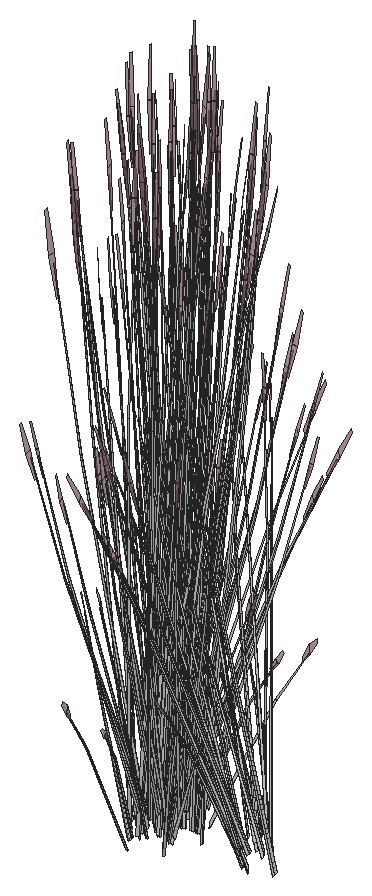
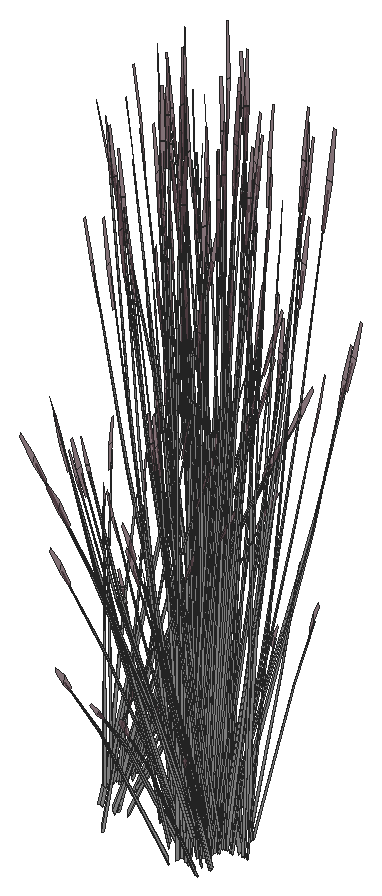
# SketchUp Ruby script. Lengths in inches.
U = 1.inch
M = Sketchup.active_model
def pt(a) = Geom::Point3d.new(a.map { |v| v * U })
def face(e, loops, mat)
  f = e.add_face(loops[0].map { |a| pt(a) })
  loops[1..].each { |l| e.add_face(l.map { |a| pt(a) }).erase! }
  f.material = f.back_material = mat if mat
  f
end
# faces: each face lists its corners as indices into pts; further lists are holes
def faces(e, pts, list, mat = nil) = list.each { |f| face(e, (f[0].is_a?(Array) ? f : [f]).map { |l| l.map { |i| pts[i] } }, mat) }
# xy, xz, yz: faces in a plane at the given z, y or x. An outline is a flat list of corners, or four numbers for a rectangle; further outlines are holes
def ring(l) = l.size == 4 ? [[l[0], l[1]], [l[2], l[1]], [l[2], l[3]], [l[0], l[3]]] : l.each_slice(2).to_a
def flat(e, list, mat, &to3) = list.each { |f| face(e, (f[0].is_a?(Array) ? f : [f]).map { |l| ring(l).map { |u, v| to3.(u, v) } }, mat) }
def xy(e, z, list, mat = nil) = flat(e, list, mat) { |x, y| [x, y, z] }
def xz(e, y, list, mat = nil) = flat(e, list, mat) { |x, z| [x, y, z] }
def yz(e, x, list, mat = nil) = flat(e, list, mat) { |y, z| [x, y, z] }
def lines(e, pts, list) = list.each { |a, b| e.add_line(pt(pts[a]), pt(pts[b])) }
# prism: a flat outline (further loops are holes) pulled along v
def prism(e, loops, v, mat = nil)
  f = face(e, loops, mat); d = Geom::Vector3d.new(v.map { |x| x * U })
  f.pushpull(f.normal.samedirection?(d) ? d.length : -d.length)
end
def box(e, o, s, mat = nil) = prism(e, [[o, [o[0] + s[0], o[1], o[2]], [o[0] + s[0], o[1] + s[1], o[2]], [o[0], o[1] + s[1], o[2]]]], [0, 0, s[2]], mat)
def at(x, y, z, deg = 0) = Geom::Transformation.translation(pt([x, y, z])) * Geom::Transformation.rotation(ORIGIN, Z_AXIS, deg.degrees)
def axes(o, x, y, z) = Geom::Transformation.new([*x, 0, *y, 0, *z, 0, *pt(o).to_a, 1])
def part(name) = M.definitions.add(name)
# library, detail: a bought-in or finely detailed component or shape, given as its bounding box
def library(name, o, s) = part(name).tap { |d| box(d.entities, o, s) }
def detail(e, o, s) = box(e.add_group.entities, o, s)
def put(e, d, t, mat = nil) = e.add_instance(d, t).tap { |i| i.material = mat if mat }
def group(e, t, mat = nil) = e.add_group.tap { |g| g.transformation = t; g.material = mat if mat }.entities
root = M.entities
M.materials.add("LightPink_Translucent").color = [144, 107, 117]
M.materials["LightPink_Translucent"].alpha = 0.75
M.materials.add("[_0053_Ivory_]").color = [200, 200, 200]
c1 = part("blade")
p = [[2.15,0.21,22],[0,0.17,0],[0.09,0.45,0],[2.18,0.31,22],[2.29,0.31,22],[0.38,0.45,0],
  [2.48,0.24,33],[2.49,0.24,33],[2.48,0.22,33]]
faces(c1.entities,p,[[0,1,2,3],[4,5,2,3],[6,3,4,7],[8,0,3,6]])
c2 = part("seeds")
p = [[0.3,-0.1,1.38],[-0.01,-0.03,1.59],[-0.01,-0.03,0.03],[0.14,-0.07,-0.07],[0.29,-0.03,3],[0.15,0.01,3.11]]
faces(c2.entities,p,[[0,1,2,3],[1,0,4,5]],"LightPink_Translucent")
c3 = part("blade with seeds")
put(c3.entities,c1,at(0,0,0))
put(c3.entities,c2,axes([2.4,0.25,30.99],[1.5799,-0.05474,1.17369],[-0.12525,1.92788,0.29478],[-0.07173,-0.02425,1.56792]))
put(root,c3,axes([458.04,103.93,128.86],[-0.36485,-0.52782,-0.44739],[0.55265,-0.37168,0.21531],[-0.11807,-0.06531,1.43643]),"[_0053_Ivory_]")
put(root,c3,axes([457.01,105.32,131.99],[-0.0158,0.58168,-0.7886],[-0.66548,-0.03907,0.09517],[-0.07023,0.24643,1.11556]),"[_0053_Ivory_]")
put(root,c3,axes([456.99,106.96,129.42],[-0.01572,-0.37392,1.1486],[0.39276,0.26669,0.84392],[-0.07724,0.17822,0.25299]),"[_0053_Ivory_]")
put(root,c3,axes([458.82,104.31,128.86],[-0.65953,0.03882,-0.44739],[-0.05964,-0.64439,0.21531],[-0.11807,0.06531,1.43643]),"[_0053_Ivory_]")
put(root,c3,axes([457.56,105.39,129.13],[0.56842,0.31443,0.49651],[-0.33976,0.56381,0],[-0.12946,-0.07161,1.57504]),"[_0053_Ivory_]")
put(root,c3,axes([456.78,106.14,130.02],[0.01334,-0.32463,1.54345],[0.60018,0.17147,0.21329],[-0.052,0.34598,0.72882]),"[_0053_Ivory_]")
put(root,c3,axes([458.09,104.23,129.09],[0.16098,-0.74515,-0.23429],[0.76326,0.12989,0.51271],[-0.13337,-0.1029,1.5644]),"[_0053_Ivory_]")
put(root,c3,axes([458.37,104.41,129.27],[-0.11717,0.56122,0.1448],[-0.57245,-0.09742,-0.41347],[-0.10418,-0.05763,1.26744]),"[_0053_Ivory_]")
put(root,c3,axes([459.51,105.97,128.67],[-0.56842,0.31443,-0.49651],[-0.33976,-0.56381,0],[-0.12946,0.07161,1.57504]),"[_0053_Ivory_]")
put(root,c3,axes([456.14,102.84,128.67],[0,-0.62885,-0.49651],[0.67951,0,0],[0,-0.14322,1.57504]),"[_0053_Ivory_]")
put(root,c3,axes([456.44,103.42,129.13],[0,0.62885,0.49651],[-0.67951,0,0],[0,-0.14322,1.57504]),"[_0053_Ivory_]")
put(root,c3,axes([459.55,105.8,128.85],[-0.37499,-0.63235,-0.05142],[0.6353,-0.35142,0.51607],[-0.15655,0.0602,1.6363]),"[_0053_Ivory_]")
put(root,c3,axes([457.14,105.52,131.66],[0.43478,0.42253,-0.5672],[-0.45929,0.37004,-0.43934],[-0.06615,0.21468,1.08528]),"[_0053_Ivory_]")
put(root,c3,axes([459.375,105.72,128.68],[-0.56663,-0.1556,-0.30978],[0.14267,-0.54795,0.30978],[-0.11423,0.06319,1.38974]),"[_0053_Ivory_]")
put(root,c3,axes([457.92,103.57,129.32],[-0.68399,-0.30005,-0.29095],[0.32934,-0.63331,-0.50002],[-0.0215,-0.15549,1.59708]),"[_0053_Ivory_]")
put(root,c3,axes([459.7,103.38,129.5],[-0.01659,-0.59209,1.41272],[0.75089,0.15348,0.59816],[-0.1776,0.32398,1.3335]),"[_0053_Ivory_]")
put(root,c3,axes([456.67,106.15,129.48],[0.55175,-0.11136,0.06507],[0.12684,0.44864,-0.86304],[-0.03498,0.22711,0.7736]),"[_0053_Ivory_]")
put(root,c3,axes([459.28,104.13,129.32],[0.07077,0.71755,-0.29095],[-0.73712,0.04339,-0.50002],[-0.1298,0.09558,1.59708]),"[_0053_Ivory_]")
put(root,c3,axes([457.61,102.93,128.75],[-0.24943,-0.64486,-0.69835],[0.71849,-0.23224,-0.18329],[-0.02757,-0.21836,1.54149]),"[_0053_Ivory_]")
put(root,c3,axes([458.74,100.91,131.33],[-0.59704,-0.15764,-0.51099],[0.20464,-0.54049,-0.3958],[-0.05475,-0.21761,0.97773]),"[_0053_Ivory_]")
put(root,c3,axes([457.64,104.91,130.53],[-0.01487,-0.24136,1.71376],[0.64429,0.16012,0.13857],[-0.03985,0.34396,0.73262]),"[_0053_Ivory_]")
put(root,c3,axes([456.4375,102.85,128.68],[0.42396,-0.39235,-0.30978],[0.42396,0.39235,0.30978],[0,-0.12637,1.38974]),"[_0053_Ivory_]")
put(root,c3,axes([458.35,100.32,128.78],[-0.4197,0.36076,-0.03893],[-0.38456,-0.39511,-0.17649],[-0.02707,-0.11196,0.58215]),"[_0053_Ivory_]")
put(root,c3,axes([458.18,103.875,129.01],[0.76764,0.13249,0.45755],[-0.15622,0.74829,0.17955],[-0.11218,-0.07226,1.58856]),"[_0053_Ivory_]")
put(root,c3,axes([457.98,103.74,129.37],[-0.29468,0.56664,0.44739],[-0.61229,-0.27271,-0.21531],[0,-0.13062,1.43643]),"[_0053_Ivory_]")
put(root,c3,axes([458.95,101.01,131.63],[-0.28988,-0.51132,-0.71045],[0.59671,-0.28496,0.08574],[-0.06778,-0.24706,1.00501]),"[_0053_Ivory_]")
put(root,c3,axes([457.77,105.07,129.13],[0.65264,-0.16691,0.17642],[0.16115,0.62115,0.35086],[-0.05821,-0.0905,1.60407]),"[_0053_Ivory_]")
put(root,c3,axes([458.61,105.17,128.85],[-0.61229,-0.28233,0],[0.29468,-0.58663,0],[0,0,1.62707]),"[_0053_Ivory_]")
put(root,c3,axes([460.03,105.875,129.03],[0.37973,0.63014,0],[-0.6353,0.35142,-0.51607],[-0.14469,0.08004,1.63711]),"[_0053_Ivory_]")
put(root,c3,axes([459.71,105.1,129.13],[0.17545,-0.62497,0.17642],[0.64204,0.17686,0.35086],[-0.11091,0.00304,1.60407]),"[_0053_Ivory_]")
put(root,c3,axes([459.41,104.27,129.27],[0.44871,0.37783,0.1448],[-0.37428,0.42627,-0.41347],[-0.10418,0.05763,1.26744]),"[_0053_Ivory_]")
put(root,c3,axes([459.25,103.81,128.95],[-0.56493,-0.54126,-0.06131],[0.56528,-0.54159,0],[-0.01973,-0.0189,1.75571]),"[_0053_Ivory_]")
put(root,c3,axes([459.4,104,129.37],[0.65953,-0.03882,0.44739],[0.05964,0.64439,-0.21531],[-0.11807,0.06531,1.43643]),"[_0053_Ivory_]")
put(root,c3,axes([459.5625,105.48,128.98],[0.76036,0.2044,0.30756],[-0.19023,0.7306,-0.36492],[-0.12585,0.09144,1.64885]),"[_0053_Ivory_]")
put(root,c3,axes([458.45,99.875,128.15],[-0.10187,0.02266,1.76342],[-0.56336,-0.25503,-0.26939],[0.00945,-0.21273,0.30037]),"[_0053_Ivory_]")
put(root,c3,axes([459.89,105.4375,129.13],[0.56842,-0.31443,0.49651],[0.33976,0.56381,0],[-0.12946,0.07161,1.57504]),"[_0053_Ivory_]")
put(root,c3,axes([459.01,100.57,131.18],[0.1831,-0.48359,-0.35414],[0.53419,0.14105,0.4572],[-0.04898,-0.1947,0.87481]),"[_0053_Ivory_]")
put(root,c3,axes([458.12,103.18,129.01],[0.26406,0.70318,0.45755],[-0.7545,0.24452,0.17955],[0.00922,-0.12921,1.58856]),"[_0053_Ivory_]")
put(root,c3,axes([457.99,103.1,128.86],[0.29468,-0.56664,-0.44739],[0.61229,0.27271,0.21531],[0,-0.13062,1.43643]),"[_0053_Ivory_]")
put(root,c3,axes([458.75,104.92,128.86],[-0.19817,-0.54216,0],[0.56587,-0.18986,0],[0,0,1.54371]),"[_0053_Ivory_]")
put(root,c3,axes([458.03,106.07,128.15],[0.09829,-0.03422,1.76342],[0.59126,0.18834,-0.26939],[0.01729,0.21228,0.30037]),"[_0053_Ivory_]")
put(root,c3,axes([458.16,106.26,131.18],[-0.1831,0.48359,-0.35414],[-0.53419,-0.14105,0.4572],[0.04898,0.1947,0.87481]),"[_0053_Ivory_]")
put(root,c3,axes([459.55,103.85,128.86],[-0.29468,0.56664,-0.44739],[-0.61229,-0.27271,0.21531],[0,0.13062,1.43643]),"[_0053_Ivory_]")
put(root,c3,axes([460.71,103.51,129.13],[-0.47719,-0.45806,0.17642],[0.48088,-0.44429,0.35086],[-0.0527,0.09355,1.60407]),"[_0053_Ivory_]")
put(root,c3,axes([459.06,103.24,128.86],[0,-0.72763,0],[0.75945,0,0],[0,0,1.79456]),"[_0053_Ivory_]")
put(root,c3,axes([458.36,103.375,129.09],[0.68433,0.30479,0.24065],[-0.32934,0.63331,0.50002],[0,-0.14599,1.60543]),"[_0053_Ivory_]")
put(root,c3,axes([459.45,103.53,128.95],[0,0.72727,-0.05637],[-0.75945,0,0],[0,0.02286,1.79368]),"[_0053_Ivory_]")
put(root,c3,axes([458.14,102.95,129.37],[-0.65953,0.03882,0.44739],[-0.05964,-0.64439,-0.21531],[0.11807,-0.06531,1.43643]),"[_0053_Ivory_]")
put(root,c3,axes([457.83,101.85,129.13],[-0.17545,0.62497,0.17642],[-0.64204,-0.17686,0.35086],[0.11091,-0.00304,1.60407]),"[_0053_Ivory_]")
put(root,c3,axes([459.08,104.94,128.94],[0.26406,0.72244,-0.06012],[-0.7545,0.25315,0],[0.00922,0.02523,1.72173]),"[_0053_Ivory_]")
put(root,c3,axes([457.52,101.07,129.03],[-0.37973,-0.63014,0],[0.6353,-0.35142,-0.51607],[0.14469,-0.08004,1.63711]),"[_0053_Ivory_]")
put(root,c3,axes([458.21,105.82,131.63],[0.28988,0.51132,-0.71045],[-0.59671,0.28496,0.08574],[0.06778,0.24706,1.00501]),"[_0053_Ivory_]")
put(root,c3,axes([461.26,103.99,128.85],[-0.75908,-0.00503,-0.04976],[0,-0.70283,0.49943],[-0.02386,0.16,1.58352]),"[_0053_Ivory_]")
put(root,c3,axes([459.77,101.88,129.13],[-0.65264,0.16691,0.17642],[-0.16115,-0.62115,0.35086],[0.05821,0.0905,1.60407]),"[_0053_Ivory_]")
put(root,c3,axes([459.11,99.55,129.42],[0.07791,0.3667,1.1486],[-0.43222,-0.2031,0.84392],[0.04651,-0.18776,0.25299]),"[_0053_Ivory_]")
put(root,c3,axes([458.7,102.79,129.01],[-0.50358,0.57069,0.45755],[-0.59827,-0.50377,0.17955],[0.1214,-0.05695,1.58856]),"[_0053_Ivory_]")
put(root,c3,axes([459.57,103.6875,128.87],[0.42396,0.40619,0],[-0.42396,0.40619,0],[0,0,1.69266]),"[_0053_Ivory_]")
put(root,c3,axes([459.56,103.21,129.37],[0.29468,-0.56664,0.44739],[0.61229,0.27271,-0.21531],[0,0.13062,1.43643]),"[_0053_Ivory_]")
put(root,c3,axes([459.3,105.18,128.86],[0.61229,0.28233,0],[-0.29468,0.58663,0],[0,0,1.74954]),"[_0053_Ivory_]")
put(root,c3,axes([458.43,105.93,131.33],[0.59704,0.15764,-0.51099],[-0.20464,0.54049,-0.3958],[0.05475,0.21761,0.97773]),"[_0053_Ivory_]")
put(root,c3,axes([459.36,103.08,129.03],[-0.76764,-0.13249,0.49198],[0.15622,-0.74829,0.19306],[0.11218,0.07226,1.70813]),"[_0053_Ivory_]")
put(root,c3,axes([461.11,104.1,128.68],[-0.42396,0.39235,-0.30978],[-0.42396,-0.39235,0.30978],[0,0.12637,1.38974]),"[_0053_Ivory_]")
put(root,c3,axes([459.89,104.02,128.75],[0.2227,0.57576,-0.69212],[-0.64151,0.20736,-0.18165],[0.02462,0.19497,1.52773]),"[_0053_Ivory_]")
put(root,c3,axes([459.58,103.41,128.86],[0.67951,0,0],[0,0.65103,0],[0,0,1.78407]),"[_0053_Ivory_]")
put(root,c3,axes([458.93,102.6875,129.37],[-0.36485,-0.52782,0.44739],[0.55265,-0.37168,-0.21531],[0.11807,0.06531,1.43643]),"[_0053_Ivory_]")
put(root,c3,axes([458.26,102.8125,129.32],[-0.07077,-0.71755,-0.29095],[0.73712,-0.04339,-0.50002],[0.1298,-0.09558,1.59708]),"[_0053_Ivory_]")
put(root,c3,axes([459.82,103.34,129.27],[0.56587,-0.18339,0.1448],[0.19817,0.52368,-0.41347],[0,0.11525,1.26744]),"[_0053_Ivory_]")
put(root,c3,axes([460.03,101.31,131.33],[-0.43478,-0.42253,-0.51099],[0.45929,-0.37004,-0.3958],[0.06615,-0.21468,0.97773]),"[_0053_Ivory_]")
put(root,c3,axes([459.62,103.38,129.32],[0.68399,0.30005,-0.29095],[-0.32934,0.63331,-0.50002],[0.0215,0.15549,1.59708]),"[_0053_Ivory_]")
put(root,c3,axes([458.17,101.23,128.68],[0.56663,0.1556,-0.30978],[-0.14267,0.54795,0.30978],[0.11423,-0.06319,1.38974]),"[_0053_Ivory_]")
put(root,c3,axes([459.74,100.57,129.24],[-0.17264,0.12729,1.43002],[-0.51703,-0.22279,-0.30754],[0.09584,-0.27707,0.61141]),"[_0053_Ivory_]")
put(root,c3,axes([467.35,101.62,130.53],[0.25192,-0.01424,1.71376],[-0.16712,0.61729,0.13857],[-0.35901,-0.03818,0.73262]),"[_0053_Ivory_]")
put(root,c3,axes([461.11,103.53,129.13],[0,-0.62885,0.49651],[0.67951,0,0],[0,0.14322,1.57504]),"[_0053_Ivory_]")
put(root,c3,axes([461.4,104.11,128.67],[0,0.62885,-0.49651],[-0.67951,0,0],[0,0.14322,1.57504]),"[_0053_Ivory_]")
put(root,c3,axes([458.03,100.98,128.67],[0.56842,-0.31443,-0.49651],[0.33976,0.56381,0],[0.12946,-0.07161,1.57504]),"[_0053_Ivory_]")
put(root,c3,axes([458.77,104.8125,130.53],[-0.13883,-0.2019,1.71376],[0.64153,-0.16998,0.13857],[0.14499,0.31697,0.73262]),"[_0053_Ivory_]")
put(root,c3,axes([459.17,102.54,129.27],[0.11717,-0.56122,0.1448],[0.57245,0.09742,-0.41347],[0.10418,0.05763,1.26744]),"[_0053_Ivory_]")
put(root,c3,axes([459.99,101.5625,129.13],[-0.56842,-0.31443,0.49651],[0.33976,-0.56381,0],[0.12946,0.07161,1.57504]),"[_0053_Ivory_]")
put(root,c3,axes([460.16,101.51,131.63],[0.0158,-0.58168,-0.71045],[0.66548,0.03907,0.08574],[0.07023,-0.24643,1.00501]),"[_0053_Ivory_]")
put(root,c3,axes([459.49,104.85,128.84],[0.63764,-0.21337,-0.19198],[0.22406,0.61462,0.00008],[0.07038,-0.02358,1.73897]),"[_0053_Ivory_]")
put(root,c3,axes([467.46,102.71,130.53],[0.21074,-0.13302,1.71376],[0.17741,0.61464,0.13857],[-0.33083,0.13891,0.73262]),"[_0053_Ivory_]")
put(root,c3,axes([466.8,103.75,129.24],[0.21107,0.05162,1.43002],[0.13604,0.52729,-0.30754],[-0.28671,0.0987,0.61141]),"[_0053_Ivory_]")
put(root,c3,axes([459.5,103.02,128.86],[0.36485,0.52782,-0.44739],[-0.55265,0.37168,0.21531],[0.11807,0.06531,1.43643]),"[_0053_Ivory_]")
put(root,c3,axes([468.67,102.07,130],[0.17264,-0.09097,1.77064],[0.05953,0.63516,0.13857],[-0.37394,0.08428,0.63284]),"[_0053_Ivory_]")
put(root,c3,axes([460.4375,101.16,131.18],[0.41095,-0.33109,-0.35414],[0.38901,0.37805,0.4572],[0.05919,-0.19208,0.87481]),"[_0053_Ivory_]")
put(root,c3,axes([460.53,105.41,129.42],[-0.34197,-0.18082,1.1486],[0.44156,-0.18372,0.84392],[0.1191,0.15563,0.25299]),"[_0053_Ivory_]")
put(root,c3,axes([459.32,105.22,129.24],[0.01072,-0.20846,1.43002],[0.51218,-0.23285,-0.30754],[0.15811,0.2495,0.61141]),"[_0053_Ivory_]")
put(root,c3,axes([458.71,102.27,128.71],[0.40909,-0.47266,-0.62353],[0.50819,0.4286,-0.16365],[0.16393,-0.11791,1.37633]),"[_0053_Ivory_]")
put(root,c3,axes([468.11,101.05,131.63],[-0.60713,-0.01514,-0.71045],[0.04078,-0.63759,0.08574],[-0.25721,-0.06729,1.00501]),"[_0053_Ivory_]")
put(root,c3,axes([467.62,101.2,129.24],[0.11858,0.17508,1.43002],[-0.27325,0.4759,-0.30754],[-0.28057,-0.11375,0.61141]),"[_0053_Ivory_]")
put(root,c3,axes([460.5,101.85,128.68],[0.14267,0.54795,-0.30978],[-0.56663,0.1556,0.30978],[0.11423,0.06319,1.38974]),"[_0053_Ivory_]")
put(root,c3,axes([461.57,103.63,129.03],[0.75945,0,0],[0,0.70283,-0.51607],[0,0.16007,1.63711]),"[_0053_Ivory_]")
put(root,c3,axes([467.13,102.15,131.18],[-0.50475,-0.17543,-0.35414],[0.14722,-0.5118,0.4572],[-0.20322,0.04693,0.87481]),"[_0053_Ivory_]")
put(root,c3,axes([467.83,100.63,130.53],[0.2256,0.10835,1.71376],[-0.46687,0.45453,0.13857],[-0.29098,-0.20505,0.73262]),"[_0053_Ivory_]")
put(root,c3,axes([459.11,102.72,129.32],[0.61322,-0.4175,-0.29095],[0.40778,0.58992,-0.50002],[0.1513,0.05991,1.59708]),"[_0053_Ivory_]")
put(root,c3,axes([460.59,106.24,129.32],[-0.38947,-0.01972,1.0506],[0.25721,-0.41888,0.58006],[0.15386,0.14882,0.8241]),"[_0053_Ivory_]")
put(root,c3,axes([467.48,102.41,131.33],[-0.16454,0.57202,-0.51099],[-0.56413,-0.19607,-0.3958],[-0.22713,0.05245,0.97773]),"[_0053_Ivory_]")
put(root,c3,axes([459.41,101.21,130.53],[-0.11309,0.21615,1.71376],[-0.47441,-0.44731,0.13857],[0.21402,-0.27879,0.73262]),"[_0053_Ivory_]")
put(root,c3,axes([467.91,101.18,131.33],[-0.44101,0.41656,-0.51099],[-0.38623,-0.44004,-0.3958],[-0.22407,-0.06338,0.97773]),"[_0053_Ivory_]")
put(root,c3,axes([467.19,102.375,128.15],[0.0154,0.09911,1.76342],[-0.31051,0.51756,-0.26939],[-0.22056,-0.02609,0.30037]),"[_0053_Ivory_]")
put(root,c3,axes([457.57,102.35,128.25],[-0.59782,0.25177,1.28929],[-0.19028,-0.72239,0.50096],[0.36709,0.01202,1.46642]),"[_0053_Ivory_]")
put(root,c3,axes([466.36,104.86,129.42],[0.25312,-0.28501,1.1486],[0.09988,0.45119,0.84392],[-0.18292,0.08079,0.25299]),"[_0053_Ivory_]")
put(root,c3,axes([459.76,105.66,131.33],[0.59932,-0.14948,-0.51099],[0.10484,0.56611,-0.3958],[0.16097,0.16223,0.97773]),"[_0053_Ivory_]")
put(root,c3,axes([460.3125,101.23,129.03],[0.37973,-0.63014,0],[0.6353,0.35142,-0.51607],[0.14469,0.08004,1.63711]),"[_0053_Ivory_]")
put(root,c3,axes([460.95,100.96,128.15],[-0.0909,-0.04954,1.76342],[-0.2335,-0.55347,-0.26939],[0.15752,-0.1502,0.30037]),"[_0053_Ivory_]")
put(root,c3,axes([467.74,100.78,131.18],[-0.34557,-0.39372,-0.35414],[0.39459,-0.37271,0.4572],[-0.20048,-0.05671,0.87481]),"[_0053_Ivory_]")
put(root,c3,axes([460.66,101.61,128.67],[0.56842,0.31443,-0.49651],[-0.33976,0.56381,0],[0.12946,0.07161,1.57504]),"[_0053_Ivory_]")
put(root,c3,axes([468.23,103.12,130.53],[0.1517,-0.19322,1.71376],[0.38303,0.52154,0.13857],[-0.26271,0.23751,0.73262]),"[_0053_Ivory_]")
put(root,c3,axes([467.32,103.625,131.18],[-0.52868,0.08987,-0.35414],[-0.1396,-0.51376,0.4572],[-0.1515,0.13799,0.87481]),"[_0053_Ivory_]")
put(root,c3,axes([460.63,106.09,128.15],[0.04425,-0.09079,1.76342],[0.55709,-0.26738,-0.26939],[0.16889,0.13839,0.30037]),"[_0053_Ivory_]")
put(root,c3,axes([460.93,102.29,131.33],[-0.15602,-0.5742,-0.51099],[0.59087,-0.10045,-0.3958],[0.16933,-0.15423,0.97773]),"[_0053_Ivory_]")
put(root,c3,axes([467.03,105.15,128.15],[0.08147,0.06283,1.76342],[0.13814,0.58211,-0.26939],[-0.18056,0.12413,0.30037]),"[_0053_Ivory_]")
put(root,c3,axes([466.91,101.73,129.42],[0.38775,-0.045,1.1486],[-0.24596,0.39648,0.84392],[-0.19161,-0.05948,0.25299]),"[_0053_Ivory_]")
put(root,c3,axes([461.97,105.25,130.58],[-0.11624,-0.52862,-0.03492],[0.54943,-0.12153,-0.15832],[0.11473,0.03351,0.52218]),"[_0053_Ivory_]")
put(root,c3,axes([459.83,102.82,128.71],[0.63179,0.1031,-0.62353],[-0.13332,0.63596,-0.16365],[0.18854,0.07706,1.37633]),"[_0053_Ivory_]")
put(root,c3,axes([462.52,103.19,128.91],[-0.37654,-0.40212,-0.06488],[0.4124,-0.36845,-0.29416],[0.11685,-0.02594,0.97024]),"[_0053_Ivory_]")
put(root,c3,axes([461.66,101.15,129.42],[-0.2023,0.32011,1.1486],[-0.17388,-0.43009,0.84392],[0.16708,-0.10777,0.25299]),"[_0053_Ivory_]")
put(root,c3,axes([468.12,103.6,130.53],[0.11309,-0.21615,1.71376],[0.47441,0.44731,0.13857],[-0.21402,0.27879,0.73262]),"[_0053_Ivory_]")
put(root,c3,axes([459.7,104.18,130.53],[-0.2256,-0.10835,1.71376],[0.46687,-0.45453,0.13857],[0.29098,0.20505,0.73262]),"[_0053_Ivory_]")
put(root,c3,axes([467.75,103.6875,131.33],[0.15602,0.5742,-0.51099],[-0.59087,0.10045,-0.3958],[-0.16933,0.15423,0.97773]),"[_0053_Ivory_]")
put(root,c3,axes([461.37,102.35,131.18],[0.52868,-0.08987,-0.35414],[0.1396,0.51376,0.4572],[0.1515,-0.13799,0.87481]),"[_0053_Ivory_]")
put(root,c3,axes([469.23,103.27,128.71],[-0.63179,-0.1031,-0.62353],[0.13332,-0.63596,-0.16365],[-0.18854,-0.07706,1.37633]),"[_0053_Ivory_]")
put(root,c3,axes([460.95,102.52,131.63],[0.31725,-0.49618,-0.71045],[0.55593,0.35263,0.08574],[0.18942,-0.17977,1.00501]),"[_0053_Ivory_]")
put(root,c3,axes([460.94,105.19,131.18],[0.34557,0.39372,-0.35414],[-0.39459,0.37271,0.4572],[0.20048,0.05671,0.87481]),"[_0053_Ivory_]")
put(root,c3,axes([469.16,100.3,131.63],[-0.51789,-0.30395,-0.71045],[0.36805,-0.53263,0.08574],[-0.18764,-0.18149,1.00501]),"[_0053_Ivory_]")
